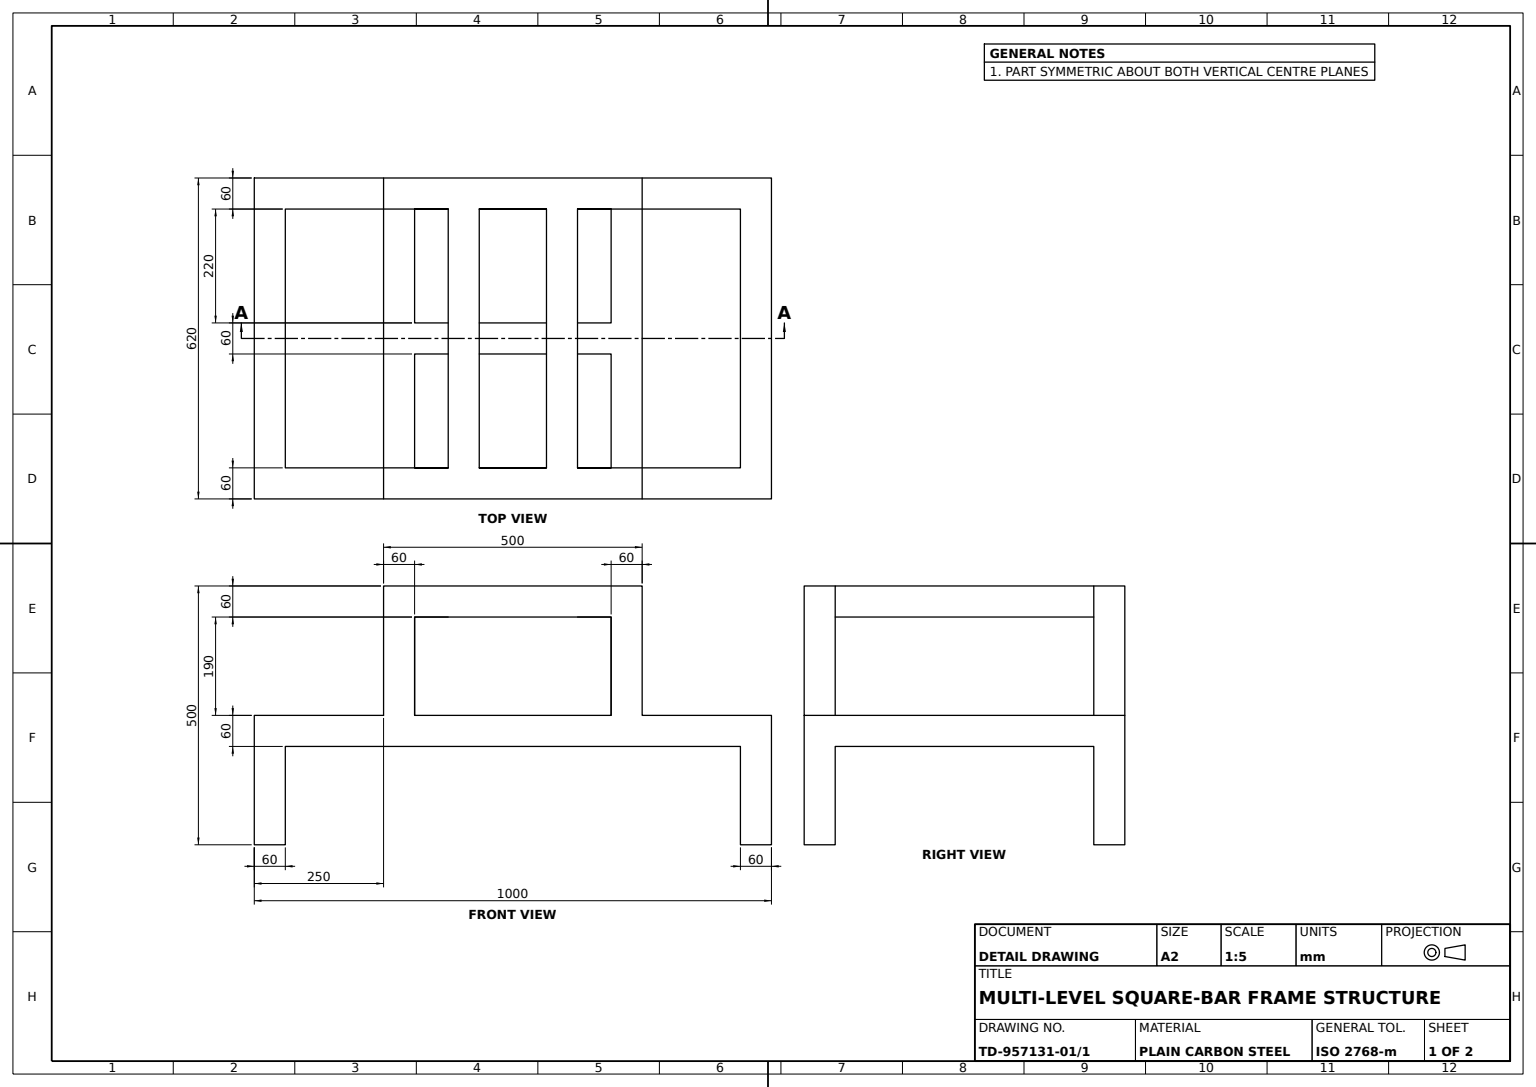
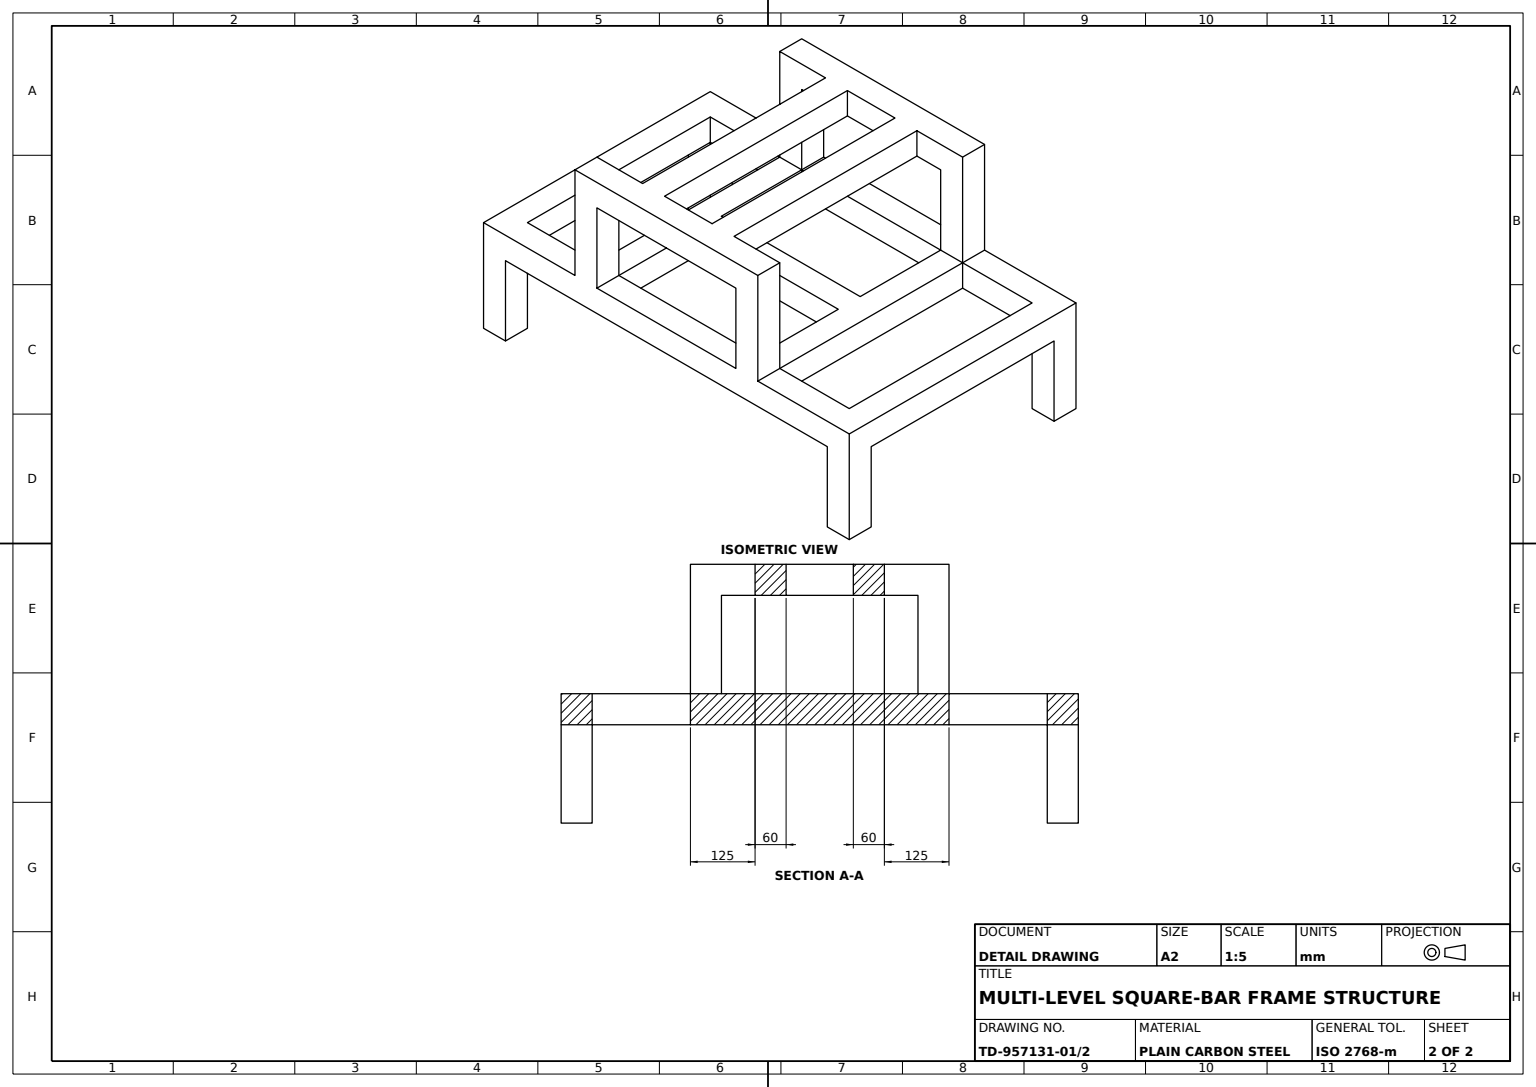
solid
v1 (1000,0,60)
v2 (1000,0,0)
e1 v1 v2 LINE
v3 (940,0,60)
e2 v3 v1 LINE
v4 (940,0,0)
e3 v3 v4 LINE
e4 v4 v2 LINE
face PLANE(AX(P(1000,0,60),D(0,1,0),D(0,0,1))) rev [-e1 -e2 e3 e4]
v5 (750,250,-500)
v6 (750,250,-560)
e5 v5 v6 LINE
v7 (750,500,-560)
e6 v7 v6 LINE
v8 (750,500,-500)
e7 v8 v7 LINE
e8 v8 v5 LINE
face PLANE(AX(P(750,250,-500),D(1,0,0),D(0,0,-1))) [e5 -e6 -e7 e8]
v9 (435,440,-500)
v10 (435,500,-500)
e9 v9 v10 LINE
v11 (565,440,-500)
e10 v11 v9 LINE
v12 (565,500,-500)
e11 v11 v12 LINE
e12 v10 v12 LINE
face PLANE(AX(P(0,0,-500),D(0,0,1),D(1,0,0))) [-e9 -e10 e11 -e12]
v13 (940,190,0)
v14 (940,250,0)
e13 v13 v14 LINE
v15 (750,190,0)
e14 v15 v13 LINE
v16 (750,250,0)
e15 v15 v16 LINE
e16 v14 v16 LINE
face PLANE(AX(P(0,0,0),D(0,0,1),D(1,0,0))) rev [-e13 -e14 e15 -e16]
v17 (310,250,-220)
v18 (690,250,-220)
e17 v17 v18 LINE
v19 (310,190,-220)
e18 v19 v17 LINE
v20 (690,190,-220)
e19 v19 v20 LINE
e20 v20 v18 LINE
face PLANE(AX(P(690,190,-220),D(0,0,1),D(1,0,0))) [-e17 -e18 e19 e20]
v21 (435,440,0)
e21 v21 v9 LINE
v22 (565,440,0)
e22 v21 v22 LINE
e23 v11 v22 LINE
v23 (690,440,-560)
v24 (310,440,-560)
e24 v23 v24 LINE
v25 (690,440,-500)
e25 v25 v23 LINE
v26 (625,440,-500)
e26 v25 v26 LINE
v27 (625,440,0)
e27 v27 v26 LINE
v28 (690,440,0)
e28 v27 v28 LINE
v29 (690,440,60)
e29 v28 v29 LINE
v30 (310,440,60)
e30 v30 v29 LINE
v31 (310,440,0)
e31 v31 v30 LINE
v32 (375,440,0)
e32 v31 v32 LINE
v33 (375,440,-500)
e33 v33 v32 LINE
v34 (310,440,-500)
e34 v33 v34 LINE
e35 v34 v24 LINE
face PLANE(AX(P(690,440,0),D(0,-1,0),D(0,0,-1))) [-e21 e22 -e23 e10] [-e24 -e25 e26 -e27 e28 e29 -e30 -e31 e32 -e33 e34 e35]
v35 (940,190,-500)
v36 (940,250,-500)
e36 v35 v36 LINE
e37 v5 v36 LINE
v37 (750,190,-500)
e38 v37 v5 LINE
e39 v35 v37 LINE
face PLANE(AX(P(0,0,-500),D(0,0,1),D(1,0,0))) [e36 -e37 -e38 -e39]
v38 (310,250,-500)
e40 v34 v38 LINE
v39 (310,250,-560)
e41 v38 v39 LINE
e42 v24 v39 LINE
face PLANE(AX(P(310,250,-500),D(1,0,0),D(0,0,-1))) [e40 e41 -e42 -e35]
v40 (250,250,-500)
v41 (250,500,-500)
e43 v40 v41 LINE
v42 (250,500,-560)
e44 v41 v42 LINE
v43 (250,250,-560)
e45 v43 v42 LINE
e46 v40 v43 LINE
face PLANE(AX(P(250,500,-500),D(-1,0,0),D(0,0,1))) [e43 e44 -e45 -e46]
v44 (0,0,-500)
v45 (0,190,-500)
e47 v44 v45 LINE
v46 (60,0,-500)
e48 v46 v44 LINE
v47 (60,190,-500)
e49 v47 v46 LINE
e50 v47 v45 LINE
face PLANE(AX(P(0,0,-500),D(0,0,1),D(1,0,0))) [-e47 -e48 -e49 e50]
v48 (310,190,-280)
v49 (310,250,-280)
e51 v48 v49 LINE
v50 (310,190,-500)
e52 v48 v50 LINE
e53 v50 v38 LINE
e54 v49 v38 LINE
face PLANE(AX(P(310,190,-500),D(1,0,0),D(0,0,-1))) [-e51 e52 e53 -e54]
v51 (60,250,-500)
e55 v47 v51 LINE
v52 (60,250,0)
e56 v52 v51 LINE
v53 (60,190,0)
e57 v53 v52 LINE
e58 v53 v47 LINE
face PLANE(AX(P(60,190,-500),D(1,0,0),D(0,0,-1))) [e55 -e56 -e57 e58]
v54 (690,190,-280)
e59 v54 v48 LINE
v55 (690,250,-280)
e60 v55 v49 LINE
e61 v54 v55 LINE
face PLANE(AX(P(310,190,-280),D(0,0,-1),D(-1,0,0))) [e59 e51 -e60 -e61]
v56 (690,250,-560)
e62 v56 v23 LINE
v57 (690,250,-500)
e63 v57 v56 LINE
e64 v57 v25 LINE
face PLANE(AX(P(690,440,-500),D(-1,0,0),D(0,0,1))) [e25 -e62 -e63 e64]
v58 (250,500,0)
v59 (250,500,60)
e65 v58 v59 LINE
v60 (750,500,60)
e66 v60 v59 LINE
v61 (750,500,0)
e67 v61 v60 LINE
v62 (625,500,0)
e68 v61 v62 LINE
v63 (625,500,-500)
e69 v62 v63 LINE
e70 v63 v8 LINE
e71 v42 v7 LINE
v64 (375,500,-500)
e72 v41 v64 LINE
v65 (375,500,0)
e73 v64 v65 LINE
e74 v65 v58 LINE
v66 (565,500,0)
e75 v12 v66 LINE
v67 (435,500,0)
e76 v66 v67 LINE
e77 v67 v10 LINE
face PLANE(AX(P(250,500,0),D(0,1,0),D(0,0,1))) [e65 -e66 -e67 e68 e69 e70 e7 -e71 -e44 e72 e73 e74] [e12 e75 e76 e77]
v68 (60,190,60)
e78 v68 v53 LINE
v69 (60,0,60)
e79 v69 v68 LINE
v70 (60,0,0)
e80 v69 v70 LINE
e81 v70 v53 LINE
face PLANE(AX(P(60,0,60),D(-1,0,0),D(0,0,1))) rev [-e78 -e79 e80 e81]
v71 (310,250,0)
e82 v71 v17 LINE
v72 (690,250,0)
e83 v18 v72 LINE
e84 v72 v16 LINE
e85 v16 v5 LINE
e86 v5 v57 LINE
e87 v57 v55 LINE
e88 v38 v40 LINE
v73 (250,250,0)
e89 v40 v73 LINE
e90 v73 v71 LINE
face PLANE(AX(P(0,250,0),D(0,-1,0),D(0,0,-1))) rev [e82 e17 e83 e84 e85 e86 e87 e60 e54 e88 e89 e90]
v74 (310,190,0)
v75 (690,190,0)
e91 v74 v75 LINE
e92 v20 v75 LINE
e93 v74 v19 LINE
v76 (250,190,0)
e94 v53 v76 LINE
v77 (250,190,-500)
e95 v77 v76 LINE
e96 v77 v47 LINE
v78 (60,190,-560)
e97 v78 v47 LINE
v79 (940,190,-560)
e98 v79 v78 LINE
e99 v79 v35 LINE
e100 v15 v37 LINE
v80 (940,190,60)
e101 v80 v13 LINE
e102 v68 v80 LINE
v81 (690,190,-500)
e103 v81 v54 LINE
e104 v81 v50 LINE
face PLANE(AX(P(940,190,60),D(0,1,0),D(0,0,1))) rev [e91 -e92 -e19 -e93] [e78 e94 -e95 e96 -e97 -e98 e99 e39 -e100 e14 -e101 -e102] [-e59 -e103 e104 -e52]
e105 v13 v4 LINE
e106 v80 v3 LINE
face PLANE(AX(P(940,0,60),D(1,0,0),D(0,0,-1))) rev [e105 -e3 -e106 e101]
e107 v81 v57 LINE
face PLANE(AX(P(690,190,0),D(-1,0,0),D(0,0,1))) [-e107 e103 e61 -e87]
v82 (0,190,0)
e108 v82 v53 LINE
v83 (0,0,0)
e109 v83 v70 LINE
e110 v82 v83 LINE
face PLANE(AX(P(0,0,0),D(0,0,1),D(1,0,0))) rev [e108 -e81 -e109 -e110]
v84 (690,250,60)
e111 v72 v84 LINE
e112 v29 v84 LINE
e113 v28 v72 LINE
face PLANE(AX(P(690,250,0),D(-1,0,0),D(0,0,1))) [e111 -e112 -e29 e113]
e114 v32 v65 LINE
e115 v33 v64 LINE
face PLANE(AX(P(375,440,-500),D(-1,0,0),D(0,0,1))) [e114 -e73 -e115 e33]
e116 v71 v31 LINE
v85 (310,250,60)
e117 v85 v30 LINE
e118 v71 v85 LINE
face PLANE(AX(P(310,440,0),D(1,0,0),D(0,0,-1))) [e116 e31 -e117 -e118]
v86 (0,0,-560)
v87 (0,250,-560)
e119 v86 v87 LINE
e120 v86 v44 LINE
e121 v45 v82 LINE
v88 (0,0,60)
e122 v88 v83 LINE
v89 (0,250,60)
e123 v89 v88 LINE
e124 v89 v87 LINE
face PLANE(AX(P(0,0,60),D(1,0,0),D(0,0,-1))) rev [-e119 e120 e47 e121 e110 -e122 -e123 e124]
v90 (750,250,60)
e125 v16 v90 LINE
e126 v16 v61 LINE
e127 v90 v60 LINE
face PLANE(AX(P(750,250,0),D(1,0,0),D(0,0,-1))) [-e125 e126 e67 -e127]
v91 (1000,250,-560)
e128 v6 v91 LINE
v92 (1000,0,-560)
e129 v91 v92 LINE
v93 (940,0,-560)
e130 v92 v93 LINE
e131 v93 v79 LINE
v94 (60,0,-560)
e132 v78 v94 LINE
e133 v94 v86 LINE
e134 v87 v43 LINE
e135 v39 v56 LINE
face PLANE(AX(P(0,0,-560),D(0,0,1),D(1,0,0))) rev [e71 e6 e128 e129 e130 e131 e98 e132 e133 e119 e134 e45] [e62 e24 e42 e135]
e136 v77 v40 LINE
e137 v76 v73 LINE
face PLANE(AX(P(250,190,0),D(-1,0,0),D(0,0,1))) [-e136 e95 e137 -e89]
e138 v22 v66 LINE
face PLANE(AX(P(565,440,-500),D(-1,0,0),D(0,0,1))) [-e75 -e11 e23 e138]
e139 v75 v72 LINE
e140 v74 v71 LINE
e141 v72 v71 LINE
face PLANE(AX(P(0,0,0),D(0,0,1),D(1,0,0))) rev [-e139 -e91 e140 -e141]
e142 v38 v57 LINE
face PLANE(AX(P(0,250,60),D(0,-1,0),D(0,0,-1))) rev [e63 -e135 -e41 e142]
v95 (940,0,-500)
e143 v93 v95 LINE
e144 v95 v35 LINE
face PLANE(AX(P(940,190,-560),D(1,0,0),D(0,0,-1))) rev [e143 e144 -e99 -e131]
e145 v51 v40 LINE
face PLANE(AX(P(0,0,-500),D(0,0,1),D(1,0,0))) [-e96 e136 -e145 -e55]
e146 v58 v73 LINE
face PLANE(AX(P(0,0,0),D(0,0,1),D(1,0,0))) rev [-e114 -e32 -e116 -e90 -e146 -e74]
v96 (250,250,60)
e147 v73 v96 LINE
e148 v59 v96 LINE
face PLANE(AX(P(250,250,0),D(-1,0,0),D(0,0,1))) [e147 -e148 -e65 e146]
e149 v27 v62 LINE
e150 v26 v63 LINE
face PLANE(AX(P(625,440,0),D(1,0,0),D(0,0,-1))) [-e69 -e149 e27 e150]
e151 v73 v52 LINE
face PLANE(AX(P(0,0,0),D(0,0,1),D(1,0,0))) rev [-e137 -e94 e57 -e151]
e152 v96 v89 LINE
face PLANE(AX(P(0,250,60),D(0,-1,0),D(0,0,-1))) rev [-e152 -e147 e151 e56 e145 e46 -e134 -e124]
v97 (1000,190,-500)
v98 (1000,0,-500)
e153 v97 v98 LINE
e154 v97 v35 LINE
e155 v98 v95 LINE
face PLANE(AX(P(0,0,-500),D(0,0,1),D(1,0,0))) [-e153 e154 -e144 -e155]
e156 v94 v46 LINE
face PLANE(AX(P(0,0,-560),D(0,1,0),D(0,0,1))) rev [-e120 -e133 e156 e48]
face PLANE(AX(P(690,190,0),D(-1,0,0),D(0,0,1))) [-e20 e92 e139 -e83]
v99 (1000,190,0)
e157 v99 v97 LINE
e158 v13 v99 LINE
e159 v35 v13 LINE
face PLANE(AX(P(0,190,0),D(0,1,0),D(0,0,1))) rev [-e157 -e158 -e159 -e154]
e160 v21 v67 LINE
face PLANE(AX(P(435,440,0),D(1,0,0),D(0,0,-1))) [-e77 -e160 e21 e9]
e161 v88 v69 LINE
face PLANE(AX(P(0,0,60),D(0,1,0),D(0,0,1))) rev [e122 e109 -e80 -e161]
e162 v2 v99 LINE
face PLANE(AX(P(0,0,0),D(0,0,1),D(1,0,0))) rev [e158 -e162 -e4 -e105]
face PLANE(AX(P(0,0,-500),D(0,0,1),D(1,0,0))) [-e64 -e86 -e8 -e70 -e150 -e26]
face PLANE(AX(P(0,0,0),D(0,0,1),D(1,0,0))) rev [e149 -e68 -e126 -e84 -e113 -e28]
e163 v92 v98 LINE
face PLANE(AX(P(940,0,-560),D(0,1,0),D(0,0,1))) rev [-e130 e163 e155 -e143]
v100 (1000,250,60)
e164 v1 v100 LINE
e165 v100 v90 LINE
e166 v84 v85 LINE
face PLANE(AX(P(0,0,60),D(0,0,1),D(1,0,0))) [e161 e79 e102 e106 e2 e164 e165 e127 e66 e148 e152 e123] [e30 e112 e166 e117]
face PLANE(AX(P(750,190,-500),D(1,0,0),D(0,0,-1))) [e38 -e85 -e15 e100]
face PLANE(AX(P(0,190,0),D(0,-1,0),D(0,0,-1))) [-e121 -e50 -e58 -e108]
face PLANE(AX(P(0,0,-500),D(0,0,1),D(1,0,0))) [-e142 -e53 -e104 e107]
e167 v36 v14 LINE
face PLANE(AX(P(940,190,-500),D(-1,0,0),D(0,0,1))) [e13 -e167 -e36 e159]
face PLANE(AX(P(0,0,0),D(0,0,1),D(1,0,0))) rev [-e138 -e22 e160 -e76]
e168 v100 v91 LINE
face PLANE(AX(P(0,250,60),D(0,-1,0),D(0,0,-1))) rev [e16 e125 -e165 e168 -e128 -e5 e37 e167]
face PLANE(AX(P(0,250,60),D(0,-1,0),D(0,0,-1))) rev [e141 e118 -e166 -e111]
face PLANE(AX(P(1000,250,60),D(-1,0,0),D(0,0,1))) rev [e1 e162 e157 e153 -e163 -e129 -e168 -e164]
face PLANE(AX(P(0,0,-500),D(0,0,1),D(1,0,0))) [-e43 -e88 -e40 -e34 e115 -e72]
face PLANE(AX(P(310,190,-500),D(1,0,0),D(0,0,-1))) [-e140 e93 e18 -e82]
face PLANE(AX(P(60,0,-560),D(-1,0,0),D(0,0,1))) rev [e97 e49 -e156 -e132]
